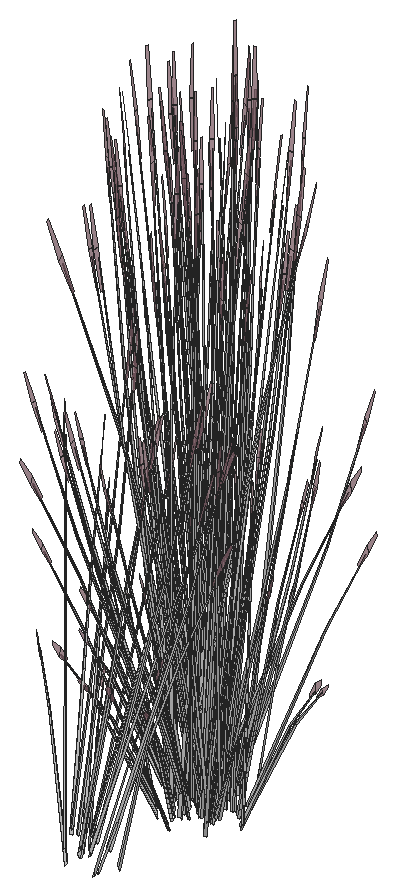
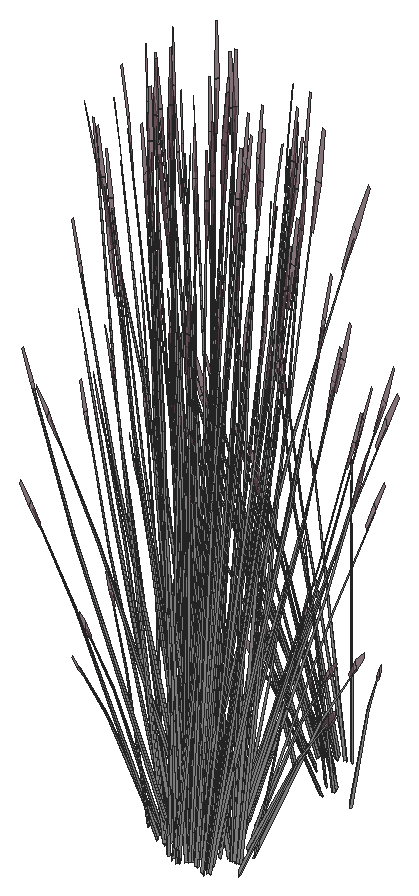
# SketchUp Ruby script. Lengths in inches.
U = 1.inch
M = Sketchup.active_model
def pt(a) = Geom::Point3d.new(a.map { |v| v * U })
def face(e, loops, mat)
  f = e.add_face(loops[0].map { |a| pt(a) })
  loops[1..].each { |l| e.add_face(l.map { |a| pt(a) }).erase! }
  f.material = f.back_material = mat if mat
  f
end
# faces: each face lists its corners as indices into pts; further lists are holes
def faces(e, pts, list, mat = nil) = list.each { |f| face(e, (f[0].is_a?(Array) ? f : [f]).map { |l| l.map { |i| pts[i] } }, mat) }
# xy, xz, yz: faces in a plane at the given z, y or x. An outline is a flat list of corners, or four numbers for a rectangle; further outlines are holes
def ring(l) = l.size == 4 ? [[l[0], l[1]], [l[2], l[1]], [l[2], l[3]], [l[0], l[3]]] : l.each_slice(2).to_a
def flat(e, list, mat, &to3) = list.each { |f| face(e, (f[0].is_a?(Array) ? f : [f]).map { |l| ring(l).map { |u, v| to3.(u, v) } }, mat) }
def xy(e, z, list, mat = nil) = flat(e, list, mat) { |x, y| [x, y, z] }
def xz(e, y, list, mat = nil) = flat(e, list, mat) { |x, z| [x, y, z] }
def yz(e, x, list, mat = nil) = flat(e, list, mat) { |y, z| [x, y, z] }
def lines(e, pts, list) = list.each { |a, b| e.add_line(pt(pts[a]), pt(pts[b])) }
# prism: a flat outline (further loops are holes) pulled along v
def prism(e, loops, v, mat = nil)
  f = face(e, loops, mat); d = Geom::Vector3d.new(v.map { |x| x * U })
  f.pushpull(f.normal.samedirection?(d) ? d.length : -d.length)
end
def box(e, o, s, mat = nil) = prism(e, [[o, [o[0] + s[0], o[1], o[2]], [o[0] + s[0], o[1] + s[1], o[2]], [o[0], o[1] + s[1], o[2]]]], [0, 0, s[2]], mat)
def at(x, y, z, deg = 0) = Geom::Transformation.translation(pt([x, y, z])) * Geom::Transformation.rotation(ORIGIN, Z_AXIS, deg.degrees)
def axes(o, x, y, z) = Geom::Transformation.new([*x, 0, *y, 0, *z, 0, *pt(o).to_a, 1])
def part(name) = M.definitions.add(name)
# library, detail: a bought-in or finely detailed component or shape, given as its bounding box
def library(name, o, s) = part(name).tap { |d| box(d.entities, o, s) }
def detail(e, o, s) = box(e.add_group.entities, o, s)
def put(e, d, t, mat = nil) = e.add_instance(d, t).tap { |i| i.material = mat if mat }
def group(e, t, mat = nil) = e.add_group.tap { |g| g.transformation = t; g.material = mat if mat }.entities
root = M.entities
M.materials.add("LightPink_Translucent").color = [144, 107, 117]
M.materials["LightPink_Translucent"].alpha = 0.75
M.materials.add("[_0053_Ivory_]").color = [200, 200, 200]
c1 = part("blade")
p = [[2.15,0.21,22],[0,0.17,0],[0.09,0.45,0],[2.18,0.31,22],[2.29,0.31,22],[0.38,0.45,0],
  [2.48,0.24,33],[2.49,0.24,33],[2.48,0.22,33]]
faces(c1.entities,p,[[0,1,2,3],[4,5,2,3],[6,3,4,7],[8,0,3,6]])
c2 = part("seeds")
p = [[0.3,-0.1,1.38],[-0.01,-0.03,1.59],[-0.01,-0.03,0.03],[0.14,-0.07,-0.07],[0.29,-0.03,3],[0.15,0.01,3.11]]
faces(c2.entities,p,[[0,1,2,3],[1,0,4,5]],"LightPink_Translucent")
c3 = part("blade with seeds")
put(c3.entities,c1,at(0,0,0))
put(c3.entities,c2,axes([2.4,0.25,30.99],[1.5799,-0.05474,1.17369],[-0.12525,1.92788,0.29478],[-0.07173,-0.02425,1.56792]))
put(root,c3,axes([640.76,112.05,128.15],[0.08147,0.06283,1.76342],[0.13814,0.58211,-0.26939],[-0.18056,0.12413,0.30037]),"[_0053_Ivory_]")
put(root,c3,axes([645,111.71,131.33],[0.59932,-0.14948,-0.51099],[0.10484,0.56611,-0.3958],[0.16097,0.16223,0.97773]),"[_0053_Ivory_]")
put(root,c3,axes([645.83,112.28,129.32],[-0.38947,-0.01972,1.0506],[0.25721,-0.41888,0.58006],[0.15386,0.14882,0.8241]),"[_0053_Ivory_]")
put(root,c3,axes([641.84,110.5,130.53],[0.11309,-0.21615,1.71376],[0.47441,0.44731,0.13857],[-0.21402,0.27879,0.73262]),"[_0053_Ivory_]")
put(root,c3,axes([644.56,111.26,129.24],[0.01072,-0.20846,1.43002],[0.51218,-0.23285,-0.30754],[0.15811,0.2495,0.61141]),"[_0053_Ivory_]")
put(root,c3,axes([641.97,111.72,131.18],[-0.41095,0.33109,-0.35414],[-0.38901,-0.37805,0.4572],[-0.05919,0.19208,0.87481]),"[_0053_Ivory_]")
put(root,c3,axes([642.24,113,129.42],[-0.01572,-0.37392,1.1486],[0.39276,0.26669,0.84392],[-0.07724,0.17822,0.25299]),"[_0053_Ivory_]")
put(root,c3,axes([643.27,112.11,128.15],[0.09829,-0.03422,1.76342],[0.59126,0.18834,-0.26939],[0.01729,0.21228,0.30037]),"[_0053_Ivory_]")
put(root,c3,axes([642.38,111.56,131.66],[0.43478,0.42253,-0.5672],[-0.45929,0.37004,-0.43934],[-0.06615,0.21468,1.08528]),"[_0053_Ivory_]")
put(root,c3,axes([641.91,112.19,129.48],[0.55175,-0.11136,0.06507],[0.12684,0.44864,-0.86304],[-0.03498,0.22711,0.7736]),"[_0053_Ivory_]")
put(root,c3,axes([643.67,111.97,131.33],[0.59704,0.15764,-0.51099],[-0.20464,0.54049,-0.3958],[0.05475,0.21761,0.97773]),"[_0053_Ivory_]")
put(root,c3,axes([644.01,110.85,130.53],[-0.13883,-0.2019,1.71376],[0.64153,-0.16998,0.13857],[0.14499,0.31697,0.73262]),"[_0053_Ivory_]")
put(root,c3,axes([643.4,112.3,131.18],[-0.1831,0.48359,-0.35414],[-0.53419,-0.14105,0.4572],[0.04898,0.1947,0.87481]),"[_0053_Ivory_]")
put(root,c3,axes([642.49,121.96,130.53],[0.13883,0.2019,1.71376],[-0.64153,0.16998,0.13857],[-0.14499,-0.31697,0.73262]),"[_0053_Ivory_]")
put(root,c3,axes([642.25,111.37,131.99],[-0.0158,0.58168,-0.7886],[-0.66548,-0.03907,0.09517],[-0.07023,0.24643,1.11556]),"[_0053_Ivory_]")
put(root,c3,axes([644.98,121.67,129.24],[-0.17264,0.12729,1.43002],[-0.51703,-0.22279,-0.30754],[0.09584,-0.27707,0.61141]),"[_0053_Ivory_]")
put(root,c3,axes([644.2,122.11,131.63],[-0.28988,-0.51132,-0.71045],[0.59671,-0.28496,0.08574],[-0.06778,-0.24706,1.00501]),"[_0053_Ivory_]")
put(root,c3,axes([642.88,110.95,130.53],[-0.01487,-0.24136,1.71376],[0.64429,0.16012,0.13857],[-0.03985,0.34396,0.73262]),"[_0053_Ivory_]")
put(root,c3,axes([642.3125,121.43,129.24],[-0.03678,0.20572,1.43002],[-0.53767,0.17221,-0.30754],[-0.12568,-0.26589,0.61141]),"[_0053_Ivory_]")
put(root,c3,axes([643.7,120.98,128.15],[-0.10187,0.02266,1.76342],[-0.56336,-0.25503,-0.26939],[0.00945,-0.21273,0.30037]),"[_0053_Ivory_]")
put(root,c3,axes([643.46,111.87,131.63],[0.28988,0.51132,-0.71045],[-0.59671,0.28496,0.08574],[0.06778,0.24706,1.00501]),"[_0053_Ivory_]")
put(root,c3,axes([641.78,112.67,129.24],[0.19166,-0.0992,1.43002],[0.4732,0.29912,-0.30754],[-0.14084,0.25882,0.61141]),"[_0053_Ivory_]")
put(root,c3,axes([645.4,122.61,131.63],[0.0158,-0.58168,-0.71045],[0.66548,0.03907,0.08574],[0.07023,-0.24643,1.00501]),"[_0053_Ivory_]")
put(root,c3,axes([644.25,121.68,131.18],[0.1831,-0.48359,-0.35414],[0.53419,0.14105,0.4572],[-0.04898,-0.1947,0.87481]),"[_0053_Ivory_]")
put(root,c3,axes([644.65,122.32,130.53],[-0.11309,0.21615,1.71376],[-0.47441,-0.44731,0.13857],[0.21402,-0.27879,0.73262]),"[_0053_Ivory_]")
put(root,c3,axes([643.98,122.01,131.33],[-0.59704,-0.15764,-0.51099],[0.20464,-0.54049,-0.3958],[-0.05475,-0.21761,0.97773]),"[_0053_Ivory_]")
put(root,c3,axes([644.35,120.66,129.42],[0.07791,0.3667,1.1486],[-0.43222,-0.2031,0.84392],[0.04651,-0.18776,0.25299]),"[_0053_Ivory_]")
put(root,c3,axes([645.27,122.42,131.33],[-0.43478,-0.42253,-0.51099],[0.45929,-0.37004,-0.3958],[0.06615,-0.21468,0.97773]),"[_0053_Ivory_]")
put(root,c3,axes([642.03,112.19,130.02],[0.01334,-0.32463,1.54345],[0.60018,0.17147,0.21329],[-0.052,0.34598,0.72882]),"[_0053_Ivory_]")
put(root,c3,axes([645.68,122.27,131.18],[0.41095,-0.33109,-0.35414],[0.38901,0.37805,0.4572],[0.05919,-0.19208,0.87481]),"[_0053_Ivory_]")
put(root,c3,axes([642.125,121.1,129.42],[0.31682,0.21887,1.1486],[-0.4614,0.13157,0.84392],[-0.09872,-0.16821,0.25299]),"[_0053_Ivory_]")
put(root,c3,axes([642.89,122.26,131.63],[-0.51789,-0.30395,-0.71045],[0.36805,-0.53263,0.08574],[-0.18764,-0.18149,1.00501]),"[_0053_Ivory_]")
put(root,c3,axes([642.71,121.86,131.18],[-0.0938,-0.50652,-0.35414],[0.53623,-0.13375,0.4572],[-0.14403,-0.14515,0.87481]),"[_0053_Ivory_]")
put(root,c3,axes([641.875,121.76,128.15],[-0.05883,0.08284,1.76342],[-0.59454,0.17861,-0.26939],[-0.14363,-0.16248,0.30037]),"[_0053_Ivory_]")
put(root,c3,axes([642.86,124.04,128.75],[-0.24943,-0.64486,-0.69835],[0.71849,-0.23224,-0.18329],[-0.02757,-0.21836,1.54149]),"[_0053_Ivory_]")
put(root,c3,axes([646.19,122.06,128.15],[-0.0909,-0.04954,1.76342],[-0.2335,-0.55347,-0.26939],[0.15752,-0.1502,0.30037]),"[_0053_Ivory_]")
put(root,c3,axes([642.65,122.28,131.33],[-0.59932,0.14948,-0.51099],[-0.10484,-0.56611,-0.3958],[-0.16097,-0.16223,0.97773]),"[_0053_Ivory_]")
put(root,c3,axes([646.1875,123.625,131.63],[0.31725,-0.49618,-0.71045],[0.55593,0.35263,0.08574],[0.18942,-0.17977,1.00501]),"[_0053_Ivory_]")
put(root,c3,axes([642.76,122.18,129.03],[-0.37973,-0.63014,0],[0.6353,-0.35142,-0.51607],[0.14469,-0.08004,1.63711]),"[_0053_Ivory_]")
put(root,c3,axes([646.17,123.39,131.33],[-0.15602,-0.5742,-0.51099],[0.59087,-0.10045,-0.3958],[0.16933,-0.15423,0.97773]),"[_0053_Ivory_]")
put(root,c3,axes([643.59,121.42,128.78],[-0.4197,0.36076,-0.03893],[-0.38456,-0.39511,-0.17649],[-0.02707,-0.11196,0.58215]),"[_0053_Ivory_]")
put(root,c3,axes([644.13,125.7,129.98],[0.52485,0.25358,1.51261],[-0.51417,0.54629,0.59816],[-0.23031,-0.32378,1.26806]),"[_0053_Ivory_]")
put(root,c3,axes([641.39,123.95,128.67],[0,-0.62885,-0.49651],[0.67951,0,0],[0,-0.14322,1.57504]),"[_0053_Ivory_]")
put(root,c3,axes([643.27,122.08,128.67],[0.56842,-0.31443,-0.49651],[0.33976,0.56381,0],[0.12946,-0.07161,1.57504]),"[_0053_Ivory_]")
put(root,c3,axes([646.65,123.17,129.24],[-0.21697,-0.01863,1.43002],[-0.22228,-0.49966,-0.30754],[0.26655,-0.14135,0.61141]),"[_0053_Ivory_]")
put(root,c3,axes([643.95,123.375,128.71],[0.40909,-0.47266,-0.62353],[0.50819,0.4286,-0.16365],[0.16393,-0.11791,1.37633]),"[_0053_Ivory_]")
put(root,c3,axes([646.9,122.25,129.42],[-0.2023,0.32011,1.1486],[-0.17388,-0.43009,0.84392],[0.16708,-0.10777,0.25299]),"[_0053_Ivory_]")
put(root,c3,axes([646.61,123.45,131.18],[0.52868,-0.08987,-0.35414],[0.1396,0.51376,0.4572],[0.1515,-0.13799,0.87481]),"[_0053_Ivory_]")
put(root,c3,axes([643.24,124.2,128.86],[0.29468,-0.56664,-0.44739],[0.61229,0.27271,0.21531],[0,-0.13062,1.43643]),"[_0053_Ivory_]")
put(root,c3,axes([641.47,122.75,131.18],[-0.34557,-0.39372,-0.35414],[0.39459,-0.37271,0.4572],[-0.20048,-0.05671,0.87481]),"[_0053_Ivory_]")
put(root,c3,axes([643.5,123.92,129.32],[-0.07077,-0.71755,-0.29095],[0.73712,-0.04339,-0.50002],[0.1298,-0.09558,1.59708]),"[_0053_Ivory_]")
put(root,c3,axes([641.68,123.96,128.68],[0.42396,-0.39235,-0.30978],[0.42396,0.39235,0.30978],[0,-0.12637,1.38974]),"[_0053_Ivory_]")
put(root,c3,axes([641.51,122.08,128.78],[-0.1752,0.51349,-0.03893],[-0.53924,-0.15795,-0.17649],[-0.08187,-0.08399,0.58215]),"[_0053_Ivory_]")
put(root,c3,axes([643.16,124.67,129.32],[-0.68399,-0.30005,-0.29095],[0.32934,-0.63331,-0.50002],[-0.0215,-0.15549,1.59708]),"[_0053_Ivory_]")
put(root,c3,axes([641.22,124.42,129.03],[-0.75945,0,0],[0,-0.70283,-0.51607],[0,-0.16007,1.63711]),"[_0053_Ivory_]")
put(root,c3,axes([643.41,122.33,128.68],[0.56663,0.1556,-0.30978],[-0.14267,0.54795,0.30978],[0.11423,-0.06319,1.38974]),"[_0053_Ivory_]")
put(root,c3,axes([641.8,124.24,128.98],[-0.56493,0.5287,0.30756],[-0.56528,-0.52313,-0.36492],[-0.01973,-0.15014,1.64885]),"[_0053_Ivory_]")
put(root,c3,axes([643.6,124.48,129.09],[0.68433,0.30479,0.24065],[-0.32934,0.63331,0.50002],[0,-0.14599,1.60543]),"[_0053_Ivory_]")
put(root,c3,axes([643.33,125.34,129.09],[0.16098,-0.74515,-0.23429],[0.76326,0.12989,0.51271],[-0.13337,-0.1029,1.5644]),"[_0053_Ivory_]")
put(root,c3,axes([640.64,123.69,129.42],[0.38775,-0.045,1.1486],[-0.24596,0.39648,0.84392],[-0.19161,-0.05948,0.25299]),"[_0053_Ivory_]")
put(root,c3,axes([643.38,124.06,129.37],[-0.65953,0.03882,0.44739],[-0.05964,-0.64439,-0.21531],[0.11807,-0.06531,1.43643]),"[_0053_Ivory_]")
put(root,c3,axes([641.68,124.53,129.13],[0,0.62885,0.49651],[-0.67951,0,0],[0,-0.14322,1.57504]),"[_0053_Ivory_]")
put(root,c3,axes([646.45,124.67,131.33],[0.16454,-0.57202,-0.51099],[0.56413,0.19607,-0.3958],[0.22713,-0.05245,0.97773]),"[_0053_Ivory_]")
put(root,c3,axes([645.55,122.34,129.03],[0.37973,-0.63014,0],[0.6353,0.35142,-0.51607],[0.14469,0.08004,1.63711]),"[_0053_Ivory_]")
put(root,c3,axes([643.28,125.04,128.86],[-0.36485,-0.52782,-0.44739],[0.55265,-0.37168,0.21531],[-0.11807,-0.06531,1.43643]),"[_0053_Ivory_]")
put(root,c3,axes([643.36,124.29,129.01],[0.26406,0.70318,0.45755],[-0.7545,0.24452,0.17955],[0.00922,-0.12921,1.58856]),"[_0053_Ivory_]")
put(root,c3,axes([647.05,124.83,128.64],[-0.39118,0.07547,1.41583],[-0.06226,-0.6007,0.08104],[0.27398,-0.09092,0.80566]),"[_0053_Ivory_]")
put(root,c3,axes([647.76,124.3,128.91],[-0.37654,-0.40212,-0.06488],[0.4124,-0.36845,-0.29416],[0.11685,-0.02594,0.97024]),"[_0053_Ivory_]")
put(root,c3,axes([643.22,124.85,129.37],[-0.29468,0.56664,0.44739],[-0.61229,-0.27271,-0.21531],[0,-0.13062,1.43643]),"[_0053_Ivory_]")
put(root,c3,axes([644.31,124.35,128.86],[0,-0.72763,0],[0.75945,0,0],[0,0,1.79456]),"[_0053_Ivory_]")
put(root,c3,axes([645.23,122.67,129.13],[-0.56842,-0.31443,0.49651],[0.33976,-0.56381,0],[0.12946,0.07161,1.57504]),"[_0053_Ivory_]")
put(root,c3,axes([646.34,124.88,131.63],[0.53369,-0.27773,-0.71045],[0.29743,0.5717,0.08574],[0.25786,-0.06494,1.00501]),"[_0053_Ivory_]")
put(root,c3,axes([642.95,125.24,128.71],[-0.63179,-0.1031,-0.62353],[0.13332,-0.63596,-0.16365],[-0.18854,-0.07706,1.37633]),"[_0053_Ivory_]")
put(root,c3,axes([643.95,123.89,129.01],[-0.50358,0.57069,0.45755],[-0.59827,-0.50377,0.17955],[0.1214,-0.05695,1.58856]),"[_0053_Ivory_]")
put(root,c3,axes([644.5,124.91,128.95],[-0.56493,-0.54126,-0.06131],[0.56528,-0.54159,0],[-0.01973,-0.0189,1.75571]),"[_0053_Ivory_]")
put(root,c3,axes([643.07,122.95,129.13],[-0.17545,0.62497,0.17642],[-0.64204,-0.17686,0.35086],[0.11091,-0.00304,1.60407]),"[_0053_Ivory_]")
put(root,c3,axes([642.81,123.46,128.25],[-0.59782,0.25177,1.28929],[-0.19028,-0.72239,0.50096],[0.36709,0.01202,1.46642]),"[_0053_Ivory_]")
put(root,c3,axes([644.41,123.65,129.27],[0.11717,-0.56122,0.1448],[0.57245,0.09742,-0.41347],[0.10418,0.05763,1.26744]),"[_0053_Ivory_]")
put(root,c3,axes([643.42,124.98,129.01],[0.76764,0.13249,0.45755],[-0.15622,0.74829,0.17955],[-0.11218,-0.07226,1.58856]),"[_0053_Ivory_]")
put(root,c3,axes([647.48,124.4375,128.15],[-0.03174,-0.09547,1.76342],[0.22015,-0.55846,-0.26939],[0.22208,-0.00803,0.30037]),"[_0053_Ivory_]")
put(root,c3,axes([640.92,124.34,128.15],[0.0154,0.09911,1.76342],[-0.31051,0.51756,-0.26939],[-0.22056,-0.02609,0.30037]),"[_0053_Ivory_]")
put(root,c3,axes([644.17,123.79,129.37],[-0.36485,-0.52782,0.44739],[0.55265,-0.37168,-0.21531],[0.11807,0.06531,1.43643]),"[_0053_Ivory_]")
put(root,c3,axes([642.28,126.21,128.68],[-0.14267,-0.54795,-0.30978],[0.56663,-0.1556,0.30978],[-0.11423,-0.06319,1.38974]),"[_0053_Ivory_]")
put(root,c3,axes([643.01,126.18,129.13],[0.65264,-0.16691,0.17642],[0.16115,0.62115,0.35086],[-0.05821,-0.0905,1.60407]),"[_0053_Ivory_]")
put(root,c3,axes([644.35,123.83,129.32],[0.61322,-0.4175,-0.29095],[0.40778,0.58992,-0.50002],[0.1513,0.05991,1.59708]),"[_0053_Ivory_]")
put(root,c3,axes([646.79,124.93,131.18],[0.50475,0.17543,-0.35414],[-0.14722,0.5118,0.4572],[0.20322,-0.04693,0.87481]),"[_0053_Ivory_]")
put(root,c3,axes([642.125,126.44,128.67],[-0.56842,-0.31443,-0.49651],[0.33976,-0.56381,0],[-0.12946,-0.07161,1.57504]),"[_0053_Ivory_]")
put(root,c3,axes([645.9,122.72,128.67],[0.56842,0.31443,-0.49651],[-0.33976,0.56381,0],[0.12946,0.07161,1.57504]),"[_0053_Ivory_]")
put(root,c3,axes([644.82,124.51,128.86],[0.67951,0,0],[0,0.65103,0],[0,0,1.78407]),"[_0053_Ivory_]")
put(root,c3,axes([643.67,125.33,129.32],[-0.61322,0.4175,-0.29095],[-0.40778,-0.58992,-0.50002],[-0.1513,-0.05991,1.59708]),"[_0053_Ivory_]")
put(root,c3,axes([645.01,122.99,129.13],[-0.65264,0.16691,0.17642],[-0.16115,-0.62115,0.35086],[0.05821,0.0905,1.60407]),"[_0053_Ivory_]")
put(root,c3,axes([645.42,124.3,130.53],[-0.25192,0.01424,1.71376],[0.16712,-0.61729,0.13857],[0.35901,0.03818,0.73262]),"[_0053_Ivory_]")
put(root,c3,axes([645.74,122.95,128.68],[0.14267,0.54795,-0.30978],[-0.56663,0.1556,0.30978],[0.11423,0.06319,1.38974]),"[_0053_Ivory_]")
put(root,c3,axes([644.6,124.18,129.03],[-0.76764,-0.13249,0.49198],[0.15622,-0.74829,0.19306],[0.11218,0.07226,1.70813]),"[_0053_Ivory_]")
put(root,c3,axes([643.99,126.03,128.86],[-0.19817,-0.54216,0],[0.56587,-0.18986,0],[0,0,1.54371]),"[_0053_Ivory_]")
put(root,c3,axes([643.61,125.52,129.27],[-0.11717,0.56122,0.1448],[-0.57245,-0.09742,-0.41347],[-0.10418,-0.05763,1.26744]),"[_0053_Ivory_]")
put(root,c3,axes([644.73,125.95,128.84],[0.63764,-0.21337,-0.19198],[0.22406,0.61462,0.00008],[0.07038,-0.02358,1.73897]),"[_0053_Ivory_]")
put(root,c3,axes([644.95,126.21,129.13],[0.17545,-0.62497,0.17642],[0.64204,0.17686,0.35086],[-0.11091,0.00304,1.60407]),"[_0053_Ivory_]")
put(root,c3,axes([644.81,124.79,128.87],[0.42396,0.40619,0],[-0.42396,0.40619,0],[0,0,1.69266]),"[_0053_Ivory_]")
put(root,c3,axes([645.95,124.62,129.13],[-0.47719,-0.45806,0.17642],[0.48088,-0.44429,0.35086],[-0.0527,0.09355,1.60407]),"[_0053_Ivory_]")
put(root,c3,axes([645.07,123.92,128.71],[0.63179,0.1031,-0.62353],[-0.13332,0.63596,-0.16365],[0.18854,0.07706,1.37633]),"[_0053_Ivory_]")
put(root,c3,axes([647.86,125.03,129.42],[-0.37526,0.10382,1.1486],[0.17664,-0.42906,0.84392],[0.19907,0.02936,0.25299]),"[_0053_Ivory_]")
put(root,c3,axes([643.85,126.27,128.85],[-0.61229,-0.28233,0],[0.29468,-0.58663,0],[0,0,1.62707]),"[_0053_Ivory_]")
put(root,c3,axes([644.36,125.52,129.12],[-0.59306,-0.50614,-0.25192],[0.49904,-0.56836,0.5513],[-0.1597,0.05921,1.68216]),"[_0053_Ivory_]")
put(root,c3,axes([642.8,126.49,129.13],[0.56842,0.31443,0.49651],[-0.33976,0.56381,0],[-0.12946,-0.07161,1.57504]),"[_0053_Ivory_]")
put(root,c3,axes([644.8,124.32,129.37],[0.29468,-0.56664,0.44739],[0.61229,0.27271,-0.21531],[0,0.13062,1.43643]),"[_0053_Ivory_]")
put(root,c3,axes([644.6875,124.64,128.95],[0,0.72727,-0.05637],[-0.75945,0,0],[0,0.02286,1.79368]),"[_0053_Ivory_]")
put(root,c3,axes([644.74,124.125,128.86],[0.36485,0.52782,-0.44739],[-0.55265,0.37168,0.21531],[0.11807,0.06531,1.43643]),"[_0053_Ivory_]")
put(root,c3,axes([647.21,126.36,130.58],[-0.11624,-0.52862,-0.03492],[0.54943,-0.12153,-0.15832],[0.11473,0.03351,0.52218]),"[_0053_Ivory_]")
put(root,c3,axes([642.47,126.82,129.03],[-0.37973,0.63014,0],[-0.6353,-0.35142,-0.51607],[-0.14469,-0.08004,1.63711]),"[_0053_Ivory_]")
put(root,c3,axes([646.35,124.63,129.13],[0,-0.62885,0.49651],[0.67951,0,0],[0,0.14322,1.57504]),"[_0053_Ivory_]")
put(root,c3,axes([644.65,125.1,129.37],[0.65953,-0.03882,0.44739],[0.05964,0.64439,-0.21531],[-0.11807,0.06531,1.43643]),"[_0053_Ivory_]")
put(root,c3,axes([645.06,124.45,129.27],[0.56587,-0.18339,0.1448],[0.19817,0.52368,-0.41347],[0,0.11525,1.26744]),"[_0053_Ivory_]")
put(root,c3,axes([644.06,125.42,128.86],[-0.65953,0.03882,-0.44739],[-0.05964,-0.64439,0.21531],[-0.11807,0.06531,1.43643]),"[_0053_Ivory_]")
put(root,c3,axes([647.16,125.72,129.24],[-0.14627,-0.15466,1.43002],[0.19032,-0.51164,-0.30754],[0.29594,0.06931,0.61141]),"[_0053_Ivory_]")
put(root,c3,axes([644.55,126.29,128.86],[0.61229,0.28233,0],[-0.29468,0.58663,0],[0,0,1.74954]),"[_0053_Ivory_]")
put(root,c3,axes([644.79,126.91,128.85],[-0.37499,-0.63235,-0.05142],[0.6353,-0.35142,0.51607],[-0.15655,0.0602,1.6363]),"[_0053_Ivory_]")
put(root,c3,axes([644.66,125.38,129.27],[0.44871,0.37783,0.1448],[-0.37428,0.42627,-0.41347],[-0.10418,0.05763,1.26744]),"[_0053_Ivory_]")
put(root,c3,axes([645.82,126.03,131.63],[0.60713,0.01514,-0.71045],[-0.04078,0.63759,0.08574],[0.25721,0.06729,1.00501]),"[_0053_Ivory_]")
put(root,c3,axes([645.13,126.54,129.13],[0.56842,-0.31443,0.49651],[0.33976,0.56381,0],[-0.12946,0.07161,1.57504]),"[_0053_Ivory_]")
put(root,c3,axes([644.32,126.05,128.94],[0.26406,0.72244,-0.06012],[-0.7545,0.25315,0],[0.00922,0.02523,1.72173]),"[_0053_Ivory_]")
put(root,c3,axes([644.62,126.83,128.68],[-0.56663,-0.1556,-0.30978],[0.14267,-0.54795,0.30978],[-0.11423,0.06319,1.38974]),"[_0053_Ivory_]")
put(root,c3,axes([646.81,124.74,129.03],[0.75945,0,0],[0,0.70283,-0.51607],[0,0.16007,1.63711]),"[_0053_Ivory_]")
put(root,c3,axes([646.51,125.1,128.85],[-0.75908,-0.00503,-0.04976],[0,-0.70283,0.49943],[-0.02386,0.16,1.58352]),"[_0053_Ivory_]")
put(root,c3,axes([644.86,124.49,129.32],[0.68399,0.30005,-0.29095],[-0.32934,0.63331,-0.50002],[0.0215,0.15549,1.59708]),"[_0053_Ivory_]")
